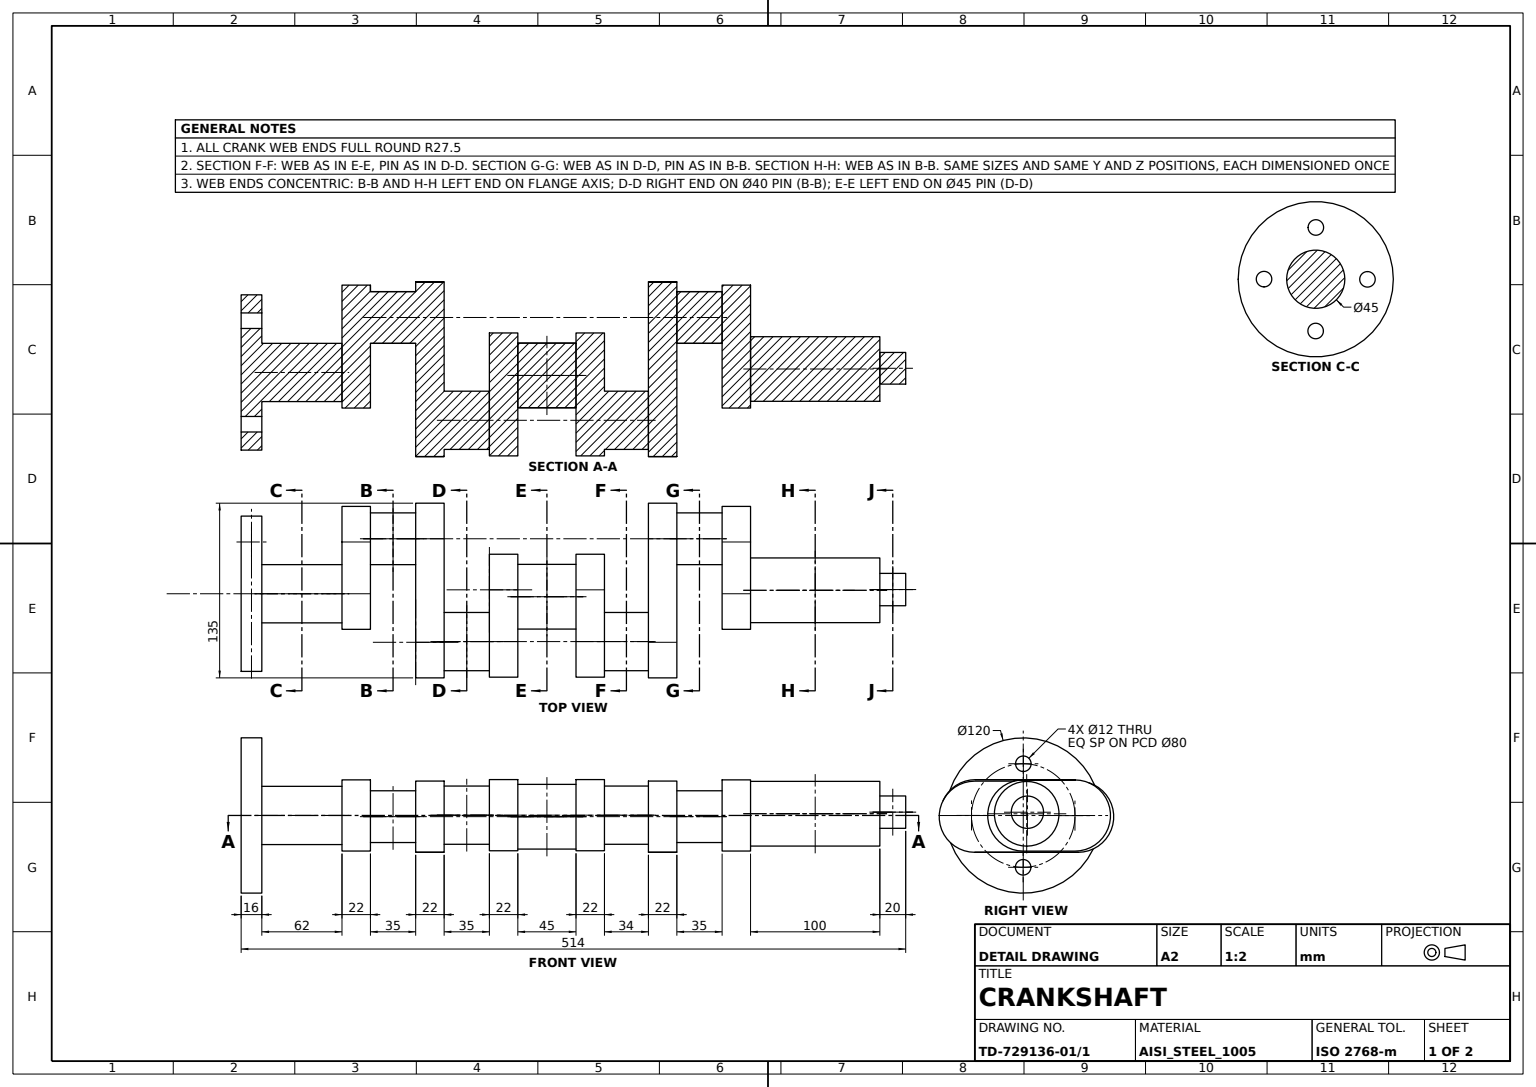
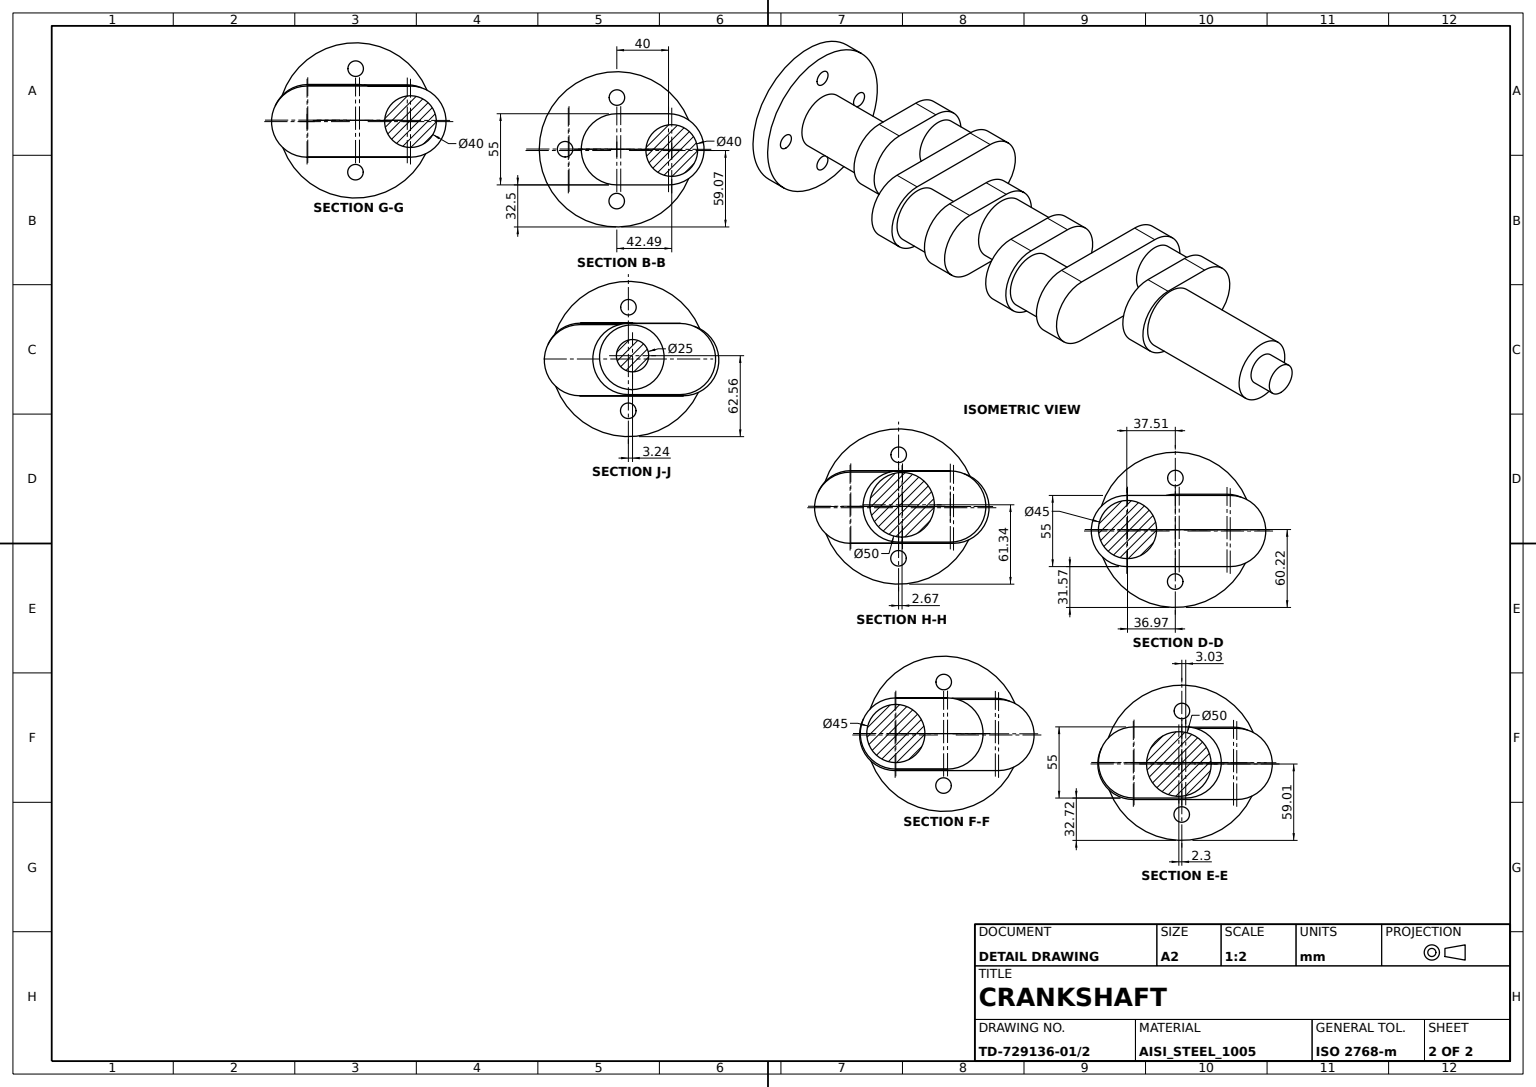
ISO-10303-21;
HEADER;
FILE_DESCRIPTION((''),'2;1');
FILE_NAME('','',(''),(''),'','','');
FILE_SCHEMA(('AUTOMOTIVE_DESIGN'));
ENDSEC;
DATA;
#1=APPLICATION_CONTEXT('');
#2=PRODUCT_CONTEXT('',#1,'mechanical');
#3=PRODUCT('','','',(#2));
#4=PRODUCT_DEFINITION_FORMATION('','',#3);
#5=PRODUCT_DEFINITION_CONTEXT('',#1,'design');
#6=PRODUCT_DEFINITION('','',#4,#5);
#7=PRODUCT_DEFINITION_SHAPE('','',#6);
#8=(LENGTH_UNIT()NAMED_UNIT(*)SI_UNIT(.MILLI.,.METRE.));
#9=(NAMED_UNIT(*)PLANE_ANGLE_UNIT()SI_UNIT($,.RADIAN.));
#10=(NAMED_UNIT(*)SI_UNIT($,.STERADIAN.)SOLID_ANGLE_UNIT());
#11=UNCERTAINTY_MEASURE_WITH_UNIT(LENGTH_MEASURE(0.005),#8,'distance_accuracy_value','');
#12=(GEOMETRIC_REPRESENTATION_CONTEXT(3)GLOBAL_UNCERTAINTY_ASSIGNED_CONTEXT((#11))GLOBAL_UNIT_ASSIGNED_CONTEXT((#8,#9,#10))REPRESENTATION_CONTEXT('',''));
#13=CARTESIAN_POINT('',(28.42745,-42.489879,-141.));
#14=VERTEX_POINT('',#13);
#15=CARTESIAN_POINT('',(-26.57255,-42.489879,-141.));
#16=VERTEX_POINT('',#15);
#17=CARTESIAN_POINT('',(0.92745,-42.489879,-141.));
#18=DIRECTION('',(0.,0.,-1.));
#19=DIRECTION('',(1.,0.,0.));
#20=AXIS2_PLACEMENT_3D('',#17,#18,#19);
#21=CIRCLE('',#20,27.5);
#22=EDGE_CURVE('',#14,#16,#21,.T.);
#23=ORIENTED_EDGE('',*,*,#22,.F.);
#24=CARTESIAN_POINT('',(28.42745,-42.489879,-119.));
#25=VERTEX_POINT('',#24);
#26=DIRECTION('',(0.,0.,1.));
#27=VECTOR('',#26,1000.);
#28=LINE('',#13,#27);
#29=EDGE_CURVE('',#14,#25,#28,.T.);
#30=ORIENTED_EDGE('',*,*,#29,.T.);
#31=CARTESIAN_POINT('',(-26.57255,-42.489879,-119.));
#32=VERTEX_POINT('',#31);
#33=CARTESIAN_POINT('',(0.92745,-42.489879,-119.));
#34=AXIS2_PLACEMENT_3D('',#33,#18,#19);
#35=CIRCLE('',#34,27.5);
#36=EDGE_CURVE('',#25,#32,#35,.T.);
#37=ORIENTED_EDGE('',*,*,#36,.T.);
#38=LINE('',#15,#27);
#39=EDGE_CURVE('',#16,#32,#38,.T.);
#40=ORIENTED_EDGE('',*,*,#39,.F.);
#41=EDGE_LOOP('',(#23,#30,#37,#40));
#42=FACE_BOUND('',#41,.T.);
#43=AXIS2_PLACEMENT_3D('',#17,#26,#19);
#44=CYLINDRICAL_SURFACE('',#43,27.5);
#45=ADVANCED_FACE('',(#42),#44,.T.);
#46=CARTESIAN_POINT('',(-26.57255,37.510121,-141.));
#47=VERTEX_POINT('',#46);
#48=CARTESIAN_POINT('',(-26.57255,37.510121,-119.));
#49=VERTEX_POINT('',#48);
#50=LINE('',#46,#27);
#51=EDGE_CURVE('',#47,#49,#50,.T.);
#52=ORIENTED_EDGE('',*,*,#51,.F.);
#53=DIRECTION('',(0.,1.,0.));
#54=VECTOR('',#53,1000.);
#55=LINE('',#15,#54);
#56=EDGE_CURVE('',#16,#47,#55,.T.);
#57=ORIENTED_EDGE('',*,*,#56,.F.);
#58=ORIENTED_EDGE('',*,*,#39,.T.);
#59=LINE('',#31,#54);
#60=EDGE_CURVE('',#32,#49,#59,.T.);
#61=ORIENTED_EDGE('',*,*,#60,.T.);
#62=EDGE_LOOP('',(#52,#57,#58,#61));
#63=FACE_BOUND('',#62,.T.);
#64=AXIS2_PLACEMENT_3D('',#15,#19,#53);
#65=PLANE('',#64);
#66=ADVANCED_FACE('',(#63),#65,.F.);
#67=ORIENTED_EDGE('',*,*,#29,.F.);
#68=CARTESIAN_POINT('',(28.42745,37.510121,-141.));
#69=VERTEX_POINT('',#68);
#70=DIRECTION('',(0.,-1.,0.));
#71=VECTOR('',#70,1000.);
#72=LINE('',#68,#71);
#73=EDGE_CURVE('',#69,#14,#72,.T.);
#74=ORIENTED_EDGE('',*,*,#73,.F.);
#75=CARTESIAN_POINT('',(28.42745,37.510121,-119.));
#76=VERTEX_POINT('',#75);
#77=LINE('',#68,#27);
#78=EDGE_CURVE('',#69,#76,#77,.T.);
#79=ORIENTED_EDGE('',*,*,#78,.T.);
#80=LINE('',#75,#71);
#81=EDGE_CURVE('',#76,#25,#80,.T.);
#82=ORIENTED_EDGE('',*,*,#81,.T.);
#83=EDGE_LOOP('',(#67,#74,#79,#82));
#84=FACE_BOUND('',#83,.T.);
#85=DIRECTION('',(-1.,0.,0.));
#86=AXIS2_PLACEMENT_3D('',#68,#85,#70);
#87=PLANE('',#86);
#88=ADVANCED_FACE('',(#84),#87,.F.);
#89=CARTESIAN_POINT('',(22.280438,36.967084,-176.));
#90=VERTEX_POINT('',#89);
#91=CARTESIAN_POINT('',(-0.219562,36.967084,-176.));
#92=AXIS2_PLACEMENT_3D('',#91,#18,#19);
#93=CIRCLE('',#92,22.5);
#94=EDGE_CURVE('',#90,#90,#93,.T.);
#95=ORIENTED_EDGE('',*,*,#94,.F.);
#96=EDGE_LOOP('',(#95));
#97=FACE_BOUND('',#96,.T.);
#98=CARTESIAN_POINT('',(22.280438,36.967084,-141.));
#99=VERTEX_POINT('',#98);
#100=CARTESIAN_POINT('',(-0.219562,36.967084,-141.));
#101=AXIS2_PLACEMENT_3D('',#100,#18,#19);
#102=CIRCLE('',#101,22.5);
#103=EDGE_CURVE('',#99,#99,#102,.T.);
#104=ORIENTED_EDGE('',*,*,#103,.T.);
#105=EDGE_LOOP('',(#104));
#106=FACE_BOUND('',#105,.T.);
#107=AXIS2_PLACEMENT_3D('',#91,#26,#19);
#108=CYLINDRICAL_SURFACE('',#107,22.5);
#109=ADVANCED_FACE('',(#97,#106),#108,.T.);
#110=CARTESIAN_POINT('',(20.92745,-42.489879,-84.));
#111=VERTEX_POINT('',#110);
#112=CARTESIAN_POINT('',(0.92745,-42.489879,-84.));
#113=AXIS2_PLACEMENT_3D('',#112,#18,#19);
#114=CIRCLE('',#113,20.);
#115=EDGE_CURVE('',#111,#111,#114,.T.);
#116=ORIENTED_EDGE('',*,*,#115,.T.);
#117=EDGE_LOOP('',(#116));
#118=FACE_BOUND('',#117,.T.);
#119=CARTESIAN_POINT('',(20.92745,-42.489879,-119.));
#120=VERTEX_POINT('',#119);
#121=CIRCLE('',#34,20.);
#122=EDGE_CURVE('',#120,#120,#121,.T.);
#123=ORIENTED_EDGE('',*,*,#122,.F.);
#124=EDGE_LOOP('',(#123));
#125=FACE_BOUND('',#124,.T.);
#126=AXIS2_PLACEMENT_3D('',#33,#26,#19);
#127=CYLINDRICAL_SURFACE('',#126,20.);
#128=ADVANCED_FACE('',(#118,#125),#127,.T.);
#129=ORIENTED_EDGE('',*,*,#122,.T.);
#130=EDGE_LOOP('',(#129));
#131=FACE_BOUND('',#130,.T.);
#132=CARTESIAN_POINT('',(0.92745,37.510121,-119.));
#133=AXIS2_PLACEMENT_3D('',#132,#18,#19);
#134=CIRCLE('',#133,27.5);
#135=EDGE_CURVE('',#49,#76,#134,.T.);
#136=ORIENTED_EDGE('',*,*,#135,.F.);
#137=ORIENTED_EDGE('',*,*,#60,.F.);
#138=ORIENTED_EDGE('',*,*,#36,.F.);
#139=ORIENTED_EDGE('',*,*,#81,.F.);
#140=EDGE_LOOP('',(#136,#137,#138,#139));
#141=FACE_BOUND('',#140,.T.);
#142=AXIS2_PLACEMENT_3D('',#132,#18,#85);
#143=PLANE('',#142);
#144=ADVANCED_FACE('',(#131,#141),#143,.F.);
#145=CARTESIAN_POINT('',(27.5,-40.,-62.));
#146=VERTEX_POINT('',#145);
#147=CARTESIAN_POINT('',(-27.5,-40.,-62.));
#148=VERTEX_POINT('',#147);
#149=CARTESIAN_POINT('',(0.,-40.,-62.));
#150=AXIS2_PLACEMENT_3D('',#149,#18,#53);
#151=CIRCLE('',#150,27.5);
#152=EDGE_CURVE('',#146,#148,#151,.T.);
#153=ORIENTED_EDGE('',*,*,#152,.F.);
#154=CARTESIAN_POINT('',(27.5,0.,-62.));
#155=VERTEX_POINT('',#154);
#156=LINE('',#154,#71);
#157=EDGE_CURVE('',#155,#146,#156,.T.);
#158=ORIENTED_EDGE('',*,*,#157,.F.);
#159=CARTESIAN_POINT('',(-27.5,0.,-62.));
#160=VERTEX_POINT('',#159);
#161=CARTESIAN_POINT('',(0.,0.,-62.));
#162=AXIS2_PLACEMENT_3D('',#161,#18,#53);
#163=CIRCLE('',#162,27.5);
#164=EDGE_CURVE('',#160,#155,#163,.T.);
#165=ORIENTED_EDGE('',*,*,#164,.F.);
#166=LINE('',#147,#54);
#167=EDGE_CURVE('',#148,#160,#166,.T.);
#168=ORIENTED_EDGE('',*,*,#167,.F.);
#169=EDGE_LOOP('',(#153,#158,#165,#168));
#170=FACE_BOUND('',#169,.T.);
#171=AXIS2_PLACEMENT_3D('',#161,#18,#85);
#172=PLANE('',#171);
#173=ADVANCED_FACE('',(#170),#172,.F.);
#174=CARTESIAN_POINT('',(27.5,-40.,-84.));
#175=VERTEX_POINT('',#174);
#176=CARTESIAN_POINT('',(-27.5,-40.,-84.));
#177=VERTEX_POINT('',#176);
#178=CARTESIAN_POINT('',(0.,-40.,-84.));
#179=AXIS2_PLACEMENT_3D('',#178,#18,#53);
#180=CIRCLE('',#179,27.5);
#181=EDGE_CURVE('',#175,#177,#180,.T.);
#182=ORIENTED_EDGE('',*,*,#181,.T.);
#183=CARTESIAN_POINT('',(-27.5,0.,-84.));
#184=VERTEX_POINT('',#183);
#185=LINE('',#176,#54);
#186=EDGE_CURVE('',#177,#184,#185,.T.);
#187=ORIENTED_EDGE('',*,*,#186,.T.);
#188=CARTESIAN_POINT('',(27.5,0.,-84.));
#189=VERTEX_POINT('',#188);
#190=CARTESIAN_POINT('',(0.,0.,-84.));
#191=AXIS2_PLACEMENT_3D('',#190,#18,#53);
#192=CIRCLE('',#191,27.5);
#193=EDGE_CURVE('',#184,#189,#192,.T.);
#194=ORIENTED_EDGE('',*,*,#193,.T.);
#195=LINE('',#188,#71);
#196=EDGE_CURVE('',#189,#175,#195,.T.);
#197=ORIENTED_EDGE('',*,*,#196,.T.);
#198=EDGE_LOOP('',(#182,#187,#194,#197));
#199=FACE_BOUND('',#198,.T.);
#200=ORIENTED_EDGE('',*,*,#115,.F.);
#201=EDGE_LOOP('',(#200));
#202=FACE_BOUND('',#201,.T.);
#203=AXIS2_PLACEMENT_3D('',#190,#18,#85);
#204=PLANE('',#203);
#205=ADVANCED_FACE('',(#199,#202),#204,.T.);
#206=ORIENTED_EDGE('',*,*,#164,.T.);
#207=LINE('',#188,#27);
#208=EDGE_CURVE('',#189,#155,#207,.T.);
#209=ORIENTED_EDGE('',*,*,#208,.F.);
#210=ORIENTED_EDGE('',*,*,#193,.F.);
#211=LINE('',#183,#27);
#212=EDGE_CURVE('',#184,#160,#211,.T.);
#213=ORIENTED_EDGE('',*,*,#212,.T.);
#214=EDGE_LOOP('',(#206,#209,#210,#213));
#215=FACE_BOUND('',#214,.T.);
#216=AXIS2_PLACEMENT_3D('',#190,#26,#19);
#217=CYLINDRICAL_SURFACE('',#216,27.5);
#218=ADVANCED_FACE('',(#215),#217,.T.);
#219=ORIENTED_EDGE('',*,*,#212,.F.);
#220=ORIENTED_EDGE('',*,*,#186,.F.);
#221=LINE('',#176,#27);
#222=EDGE_CURVE('',#177,#148,#221,.T.);
#223=ORIENTED_EDGE('',*,*,#222,.T.);
#224=ORIENTED_EDGE('',*,*,#167,.T.);
#225=EDGE_LOOP('',(#219,#220,#223,#224));
#226=FACE_BOUND('',#225,.T.);
#227=AXIS2_PLACEMENT_3D('',#176,#19,#18);
#228=PLANE('',#227);
#229=ADVANCED_FACE('',(#226),#228,.F.);
#230=LINE('',#174,#27);
#231=EDGE_CURVE('',#175,#146,#230,.T.);
#232=ORIENTED_EDGE('',*,*,#231,.F.);
#233=ORIENTED_EDGE('',*,*,#196,.F.);
#234=ORIENTED_EDGE('',*,*,#208,.T.);
#235=ORIENTED_EDGE('',*,*,#157,.T.);
#236=EDGE_LOOP('',(#232,#233,#234,#235));
#237=FACE_BOUND('',#236,.T.);
#238=AXIS2_PLACEMENT_3D('',#188,#85,#26);
#239=PLANE('',#238);
#240=ADVANCED_FACE('',(#237),#239,.F.);
#241=ORIENTED_EDGE('',*,*,#94,.T.);
#242=EDGE_LOOP('',(#241));
#243=FACE_BOUND('',#242,.T.);
#244=AXIS2_PLACEMENT_3D('',#91,#18,#85);
#245=PLANE('',#244);
#246=ADVANCED_FACE('',(#243),#245,.T.);
#247=ORIENTED_EDGE('',*,*,#152,.T.);
#248=ORIENTED_EDGE('',*,*,#222,.F.);
#249=ORIENTED_EDGE('',*,*,#181,.F.);
#250=ORIENTED_EDGE('',*,*,#231,.T.);
#251=EDGE_LOOP('',(#247,#248,#249,#250));
#252=FACE_BOUND('',#251,.T.);
#253=AXIS2_PLACEMENT_3D('',#178,#26,#19);
#254=CYLINDRICAL_SURFACE('',#253,27.5);
#255=ADVANCED_FACE('',(#252),#254,.T.);
#256=CARTESIAN_POINT('',(0.92745,37.510121,-141.));
#257=AXIS2_PLACEMENT_3D('',#256,#18,#19);
#258=CIRCLE('',#257,27.5);
#259=EDGE_CURVE('',#47,#69,#258,.T.);
#260=ORIENTED_EDGE('',*,*,#259,.F.);
#261=ORIENTED_EDGE('',*,*,#51,.T.);
#262=ORIENTED_EDGE('',*,*,#135,.T.);
#263=ORIENTED_EDGE('',*,*,#78,.F.);
#264=EDGE_LOOP('',(#260,#261,#262,#263));
#265=FACE_BOUND('',#264,.T.);
#266=AXIS2_PLACEMENT_3D('',#256,#26,#19);
#267=CYLINDRICAL_SURFACE('',#266,27.5);
#268=ADVANCED_FACE('',(#265),#267,.T.);
#269=ORIENTED_EDGE('',*,*,#22,.T.);
#270=ORIENTED_EDGE('',*,*,#56,.T.);
#271=ORIENTED_EDGE('',*,*,#259,.T.);
#272=ORIENTED_EDGE('',*,*,#73,.T.);
#273=EDGE_LOOP('',(#269,#270,#271,#272));
#274=FACE_BOUND('',#273,.T.);
#275=ORIENTED_EDGE('',*,*,#103,.F.);
#276=EDGE_LOOP('',(#275));
#277=FACE_BOUND('',#276,.T.);
#278=AXIS2_PLACEMENT_3D('',#256,#18,#85);
#279=PLANE('',#278);
#280=ADVANCED_FACE('',(#274,#277),#279,.T.);
#281=CLOSED_SHELL('',(#45,#66,#88,#109,#128,#144,#173,#205,#218,#229,#240,#246,#255,#268,#280));
#282=MANIFOLD_SOLID_BREP('',#281);
#283=CARTESIAN_POINT('',(23.658853,-2.674928,-478.));
#284=VERTEX_POINT('',#283);
#285=CARTESIAN_POINT('',(-1.341147,-2.674928,-478.));
#286=AXIS2_PLACEMENT_3D('',#285,#18,#19);
#287=CIRCLE('',#286,25.);
#288=EDGE_CURVE('',#284,#284,#287,.T.);
#289=ORIENTED_EDGE('',*,*,#288,.F.);
#290=EDGE_LOOP('',(#289));
#291=FACE_BOUND('',#290,.T.);
#292=CARTESIAN_POINT('',(23.658853,-2.674928,-378.));
#293=VERTEX_POINT('',#292);
#294=CARTESIAN_POINT('',(-1.341147,-2.674928,-378.));
#295=AXIS2_PLACEMENT_3D('',#294,#18,#19);
#296=CIRCLE('',#295,25.);
#297=EDGE_CURVE('',#293,#293,#296,.T.);
#298=ORIENTED_EDGE('',*,*,#297,.T.);
#299=EDGE_LOOP('',(#298));
#300=FACE_BOUND('',#299,.T.);
#301=AXIS2_PLACEMENT_3D('',#285,#26,#19);
#302=CYLINDRICAL_SURFACE('',#301,25.);
#303=ADVANCED_FACE('',(#291,#300),#302,.T.);
#304=ORIENTED_EDGE('',*,*,#297,.F.);
#305=EDGE_LOOP('',(#304));
#306=FACE_BOUND('',#305,.T.);
#307=AXIS2_PLACEMENT_3D('',#294,#18,#85);
#308=PLANE('',#307);
#309=ADVANCED_FACE('',(#306),#308,.F.);
#310=ORIENTED_EDGE('',*,*,#288,.T.);
#311=EDGE_LOOP('',(#310));
#312=FACE_BOUND('',#311,.T.);
#313=AXIS2_PLACEMENT_3D('',#285,#18,#85);
#314=PLANE('',#313);
#315=ADVANCED_FACE('',(#312),#314,.T.);
#316=CLOSED_SHELL('',(#303,#309,#315));
#317=MANIFOLD_SOLID_BREP('',#316);
#318=CARTESIAN_POINT('',(9.940539,-3.236305,-478.));
#319=VERTEX_POINT('',#318);
#320=CARTESIAN_POINT('',(-2.559461,-3.236305,-478.));
#321=AXIS2_PLACEMENT_3D('',#320,#18,#19);
#322=CIRCLE('',#321,12.5);
#323=EDGE_CURVE('',#319,#319,#322,.T.);
#324=ORIENTED_EDGE('',*,*,#323,.F.);
#325=EDGE_LOOP('',(#324));
#326=FACE_BOUND('',#325,.T.);
#327=AXIS2_PLACEMENT_3D('',#320,#18,#85);
#328=PLANE('',#327);
#329=ADVANCED_FACE('',(#326),#328,.F.);
#330=ORIENTED_EDGE('',*,*,#323,.T.);
#331=EDGE_LOOP('',(#330));
#332=FACE_BOUND('',#331,.T.);
#333=CARTESIAN_POINT('',(9.940539,-3.236305,-498.));
#334=VERTEX_POINT('',#333);
#335=CARTESIAN_POINT('',(-2.559461,-3.236305,-498.));
#336=AXIS2_PLACEMENT_3D('',#335,#18,#19);
#337=CIRCLE('',#336,12.5);
#338=EDGE_CURVE('',#334,#334,#337,.T.);
#339=ORIENTED_EDGE('',*,*,#338,.F.);
#340=EDGE_LOOP('',(#339));
#341=FACE_BOUND('',#340,.T.);
#342=AXIS2_PLACEMENT_3D('',#335,#26,#19);
#343=CYLINDRICAL_SURFACE('',#342,12.5);
#344=ADVANCED_FACE('',(#332,#341),#343,.T.);
#345=ORIENTED_EDGE('',*,*,#338,.T.);
#346=EDGE_LOOP('',(#345));
#347=FACE_BOUND('',#346,.T.);
#348=AXIS2_PLACEMENT_3D('',#335,#18,#85);
#349=PLANE('',#348);
#350=ADVANCED_FACE('',(#347),#349,.T.);
#351=CLOSED_SHELL('',(#329,#344,#350));
#352=MANIFOLD_SOLID_BREP('',#351);
#353=CARTESIAN_POINT('',(-39.999919,5.919571,0.));
#354=VERTEX_POINT('',#353);
#355=CARTESIAN_POINT('',(-39.999919,-0.080429,0.));
#356=AXIS2_PLACEMENT_3D('',#355,#26,#53);
#357=CIRCLE('',#356,6.);
#358=EDGE_CURVE('',#354,#354,#357,.T.);
#359=ORIENTED_EDGE('',*,*,#358,.F.);
#360=EDGE_LOOP('',(#359));
#361=FACE_BOUND('',#360,.T.);
#362=CARTESIAN_POINT('',(-39.999919,5.919571,16.));
#363=VERTEX_POINT('',#362);
#364=CARTESIAN_POINT('',(-39.999919,-0.080429,16.));
#365=AXIS2_PLACEMENT_3D('',#364,#26,#53);
#366=CIRCLE('',#365,6.);
#367=EDGE_CURVE('',#363,#363,#366,.T.);
#368=ORIENTED_EDGE('',*,*,#367,.T.);
#369=EDGE_LOOP('',(#368));
#370=FACE_BOUND('',#369,.T.);
#371=AXIS2_PLACEMENT_3D('',#364,#18,#85);
#372=CYLINDRICAL_SURFACE('',#371,6.);
#373=ADVANCED_FACE('',(#361,#370),#372,.F.);
#374=CARTESIAN_POINT('',(39.999919,-5.919571,16.));
#375=VERTEX_POINT('',#374);
#376=CARTESIAN_POINT('',(39.999919,0.080429,16.));
#377=AXIS2_PLACEMENT_3D('',#376,#26,#70);
#378=CIRCLE('',#377,6.);
#379=EDGE_CURVE('',#375,#375,#378,.T.);
#380=ORIENTED_EDGE('',*,*,#379,.F.);
#381=EDGE_LOOP('',(#380));
#382=FACE_BOUND('',#381,.T.);
#383=CARTESIAN_POINT('',(5.919571,39.999919,16.));
#384=VERTEX_POINT('',#383);
#385=CARTESIAN_POINT('',(-0.080429,39.999919,16.));
#386=AXIS2_PLACEMENT_3D('',#385,#26,#19);
#387=CIRCLE('',#386,6.);
#388=EDGE_CURVE('',#384,#384,#387,.T.);
#389=ORIENTED_EDGE('',*,*,#388,.F.);
#390=EDGE_LOOP('',(#389));
#391=FACE_BOUND('',#390,.T.);
#392=CARTESIAN_POINT('',(-5.919571,-39.999919,16.));
#393=VERTEX_POINT('',#392);
#394=CARTESIAN_POINT('',(0.080429,-39.999919,16.));
#395=AXIS2_PLACEMENT_3D('',#394,#26,#85);
#396=CIRCLE('',#395,6.);
#397=EDGE_CURVE('',#393,#393,#396,.T.);
#398=ORIENTED_EDGE('',*,*,#397,.F.);
#399=EDGE_LOOP('',(#398));
#400=FACE_BOUND('',#399,.T.);
#401=CARTESIAN_POINT('',(0.,60.,16.));
#402=VERTEX_POINT('',#401);
#403=CARTESIAN_POINT('',(0.,0.,16.));
#404=AXIS2_PLACEMENT_3D('',#403,#26,#53);
#405=CIRCLE('',#404,60.);
#406=EDGE_CURVE('',#402,#402,#405,.T.);
#407=ORIENTED_EDGE('',*,*,#406,.T.);
#408=EDGE_LOOP('',(#407));
#409=FACE_BOUND('',#408,.T.);
#410=ORIENTED_EDGE('',*,*,#367,.F.);
#411=EDGE_LOOP('',(#410));
#412=FACE_BOUND('',#411,.T.);
#413=AXIS2_PLACEMENT_3D('',#403,#26,#19);
#414=PLANE('',#413);
#415=ADVANCED_FACE('',(#382,#391,#400,#409,#412),#414,.T.);
#416=CARTESIAN_POINT('',(-5.919571,-39.999919,0.));
#417=VERTEX_POINT('',#416);
#418=CARTESIAN_POINT('',(0.080429,-39.999919,0.));
#419=AXIS2_PLACEMENT_3D('',#418,#26,#85);
#420=CIRCLE('',#419,6.);
#421=EDGE_CURVE('',#417,#417,#420,.T.);
#422=ORIENTED_EDGE('',*,*,#421,.F.);
#423=EDGE_LOOP('',(#422));
#424=FACE_BOUND('',#423,.T.);
#425=ORIENTED_EDGE('',*,*,#397,.T.);
#426=EDGE_LOOP('',(#425));
#427=FACE_BOUND('',#426,.T.);
#428=AXIS2_PLACEMENT_3D('',#394,#18,#85);
#429=CYLINDRICAL_SURFACE('',#428,6.);
#430=ADVANCED_FACE('',(#424,#427),#429,.F.);
#431=CARTESIAN_POINT('',(0.,22.5,0.));
#432=VERTEX_POINT('',#431);
#433=CARTESIAN_POINT('',(0.,0.,0.));
#434=AXIS2_PLACEMENT_3D('',#433,#18,#53);
#435=CIRCLE('',#434,22.5);
#436=EDGE_CURVE('',#432,#432,#435,.T.);
#437=ORIENTED_EDGE('',*,*,#436,.T.);
#438=EDGE_LOOP('',(#437));
#439=FACE_BOUND('',#438,.T.);
#440=CARTESIAN_POINT('',(0.,22.5,-62.));
#441=VERTEX_POINT('',#440);
#442=CIRCLE('',#162,22.5);
#443=EDGE_CURVE('',#441,#441,#442,.T.);
#444=ORIENTED_EDGE('',*,*,#443,.F.);
#445=EDGE_LOOP('',(#444));
#446=FACE_BOUND('',#445,.T.);
#447=AXIS2_PLACEMENT_3D('',#161,#26,#19);
#448=CYLINDRICAL_SURFACE('',#447,22.5);
#449=ADVANCED_FACE('',(#439,#446),#448,.T.);
#450=CARTESIAN_POINT('',(5.919571,39.999919,0.));
#451=VERTEX_POINT('',#450);
#452=CARTESIAN_POINT('',(-0.080429,39.999919,0.));
#453=AXIS2_PLACEMENT_3D('',#452,#26,#19);
#454=CIRCLE('',#453,6.);
#455=EDGE_CURVE('',#451,#451,#454,.T.);
#456=ORIENTED_EDGE('',*,*,#455,.F.);
#457=EDGE_LOOP('',(#456));
#458=FACE_BOUND('',#457,.T.);
#459=ORIENTED_EDGE('',*,*,#388,.T.);
#460=EDGE_LOOP('',(#459));
#461=FACE_BOUND('',#460,.T.);
#462=AXIS2_PLACEMENT_3D('',#385,#18,#85);
#463=CYLINDRICAL_SURFACE('',#462,6.);
#464=ADVANCED_FACE('',(#458,#461),#463,.F.);
#465=CARTESIAN_POINT('',(0.,60.,0.));
#466=VERTEX_POINT('',#465);
#467=AXIS2_PLACEMENT_3D('',#433,#26,#53);
#468=CIRCLE('',#467,60.);
#469=EDGE_CURVE('',#466,#466,#468,.T.);
#470=ORIENTED_EDGE('',*,*,#469,.T.);
#471=EDGE_LOOP('',(#470));
#472=FACE_BOUND('',#471,.T.);
#473=ORIENTED_EDGE('',*,*,#406,.F.);
#474=EDGE_LOOP('',(#473));
#475=FACE_BOUND('',#474,.T.);
#476=AXIS2_PLACEMENT_3D('',#403,#18,#85);
#477=CYLINDRICAL_SURFACE('',#476,60.);
#478=ADVANCED_FACE('',(#472,#475),#477,.T.);
#479=ORIENTED_EDGE('',*,*,#443,.T.);
#480=EDGE_LOOP('',(#479));
#481=FACE_BOUND('',#480,.T.);
#482=ADVANCED_FACE('',(#481),#172,.T.);
#483=CARTESIAN_POINT('',(39.999919,-5.919571,0.));
#484=VERTEX_POINT('',#483);
#485=CARTESIAN_POINT('',(39.999919,0.080429,0.));
#486=AXIS2_PLACEMENT_3D('',#485,#26,#70);
#487=CIRCLE('',#486,6.);
#488=EDGE_CURVE('',#484,#484,#487,.T.);
#489=ORIENTED_EDGE('',*,*,#488,.F.);
#490=EDGE_LOOP('',(#489));
#491=FACE_BOUND('',#490,.T.);
#492=ORIENTED_EDGE('',*,*,#379,.T.);
#493=EDGE_LOOP('',(#492));
#494=FACE_BOUND('',#493,.T.);
#495=AXIS2_PLACEMENT_3D('',#376,#18,#85);
#496=CYLINDRICAL_SURFACE('',#495,6.);
#497=ADVANCED_FACE('',(#491,#494),#496,.F.);
#498=ORIENTED_EDGE('',*,*,#469,.F.);
#499=EDGE_LOOP('',(#498));
#500=FACE_BOUND('',#499,.T.);
#501=ORIENTED_EDGE('',*,*,#358,.T.);
#502=EDGE_LOOP('',(#501));
#503=FACE_BOUND('',#502,.T.);
#504=ORIENTED_EDGE('',*,*,#455,.T.);
#505=EDGE_LOOP('',(#504));
#506=FACE_BOUND('',#505,.T.);
#507=ORIENTED_EDGE('',*,*,#436,.F.);
#508=EDGE_LOOP('',(#507));
#509=FACE_BOUND('',#508,.T.);
#510=ORIENTED_EDGE('',*,*,#488,.T.);
#511=EDGE_LOOP('',(#510));
#512=FACE_BOUND('',#511,.T.);
#513=ORIENTED_EDGE('',*,*,#421,.T.);
#514=EDGE_LOOP('',(#513));
#515=FACE_BOUND('',#514,.T.);
#516=AXIS2_PLACEMENT_3D('',#433,#26,#19);
#517=PLANE('',#516);
#518=ADVANCED_FACE('',(#500,#503,#506,#509,#512,#515),#517,.F.);
#519=CLOSED_SHELL('',(#373,#415,#430,#449,#464,#478,#482,#497,#518));
#520=MANIFOLD_SOLID_BREP('',#519);
#521=CARTESIAN_POINT('',(-27.719562,36.967084,-198.));
#522=VERTEX_POINT('',#521);
#523=CARTESIAN_POINT('',(-27.719562,36.967084,-176.));
#524=VERTEX_POINT('',#523);
#525=LINE('',#521,#27);
#526=EDGE_CURVE('',#522,#524,#525,.T.);
#527=ORIENTED_EDGE('',*,*,#526,.T.);
#528=CARTESIAN_POINT('',(27.280438,36.967084,-176.));
#529=VERTEX_POINT('',#528);
#530=CIRCLE('',#92,27.5);
#531=EDGE_CURVE('',#524,#529,#530,.T.);
#532=ORIENTED_EDGE('',*,*,#531,.T.);
#533=CARTESIAN_POINT('',(27.280438,36.967084,-198.));
#534=VERTEX_POINT('',#533);
#535=LINE('',#533,#27);
#536=EDGE_CURVE('',#534,#529,#535,.T.);
#537=ORIENTED_EDGE('',*,*,#536,.F.);
#538=CARTESIAN_POINT('',(-0.219562,36.967084,-198.));
#539=AXIS2_PLACEMENT_3D('',#538,#18,#19);
#540=CIRCLE('',#539,27.5);
#541=EDGE_CURVE('',#522,#534,#540,.T.);
#542=ORIENTED_EDGE('',*,*,#541,.F.);
#543=EDGE_LOOP('',(#527,#532,#537,#542));
#544=FACE_BOUND('',#543,.T.);
#545=AXIS2_PLACEMENT_3D('',#538,#26,#19);
#546=CYLINDRICAL_SURFACE('',#545,27.5);
#547=ADVANCED_FACE('',(#544),#546,.T.);
#548=ORIENTED_EDGE('',*,*,#541,.T.);
#549=CARTESIAN_POINT('',(27.280438,-3.032916,-198.));
#550=VERTEX_POINT('',#549);
#551=LINE('',#533,#71);
#552=EDGE_CURVE('',#534,#550,#551,.T.);
#553=ORIENTED_EDGE('',*,*,#552,.T.);
#554=CARTESIAN_POINT('',(-27.719562,-3.032916,-198.));
#555=VERTEX_POINT('',#554);
#556=CARTESIAN_POINT('',(-0.219562,-3.032916,-198.));
#557=AXIS2_PLACEMENT_3D('',#556,#18,#19);
#558=CIRCLE('',#557,27.5);
#559=EDGE_CURVE('',#550,#555,#558,.T.);
#560=ORIENTED_EDGE('',*,*,#559,.T.);
#561=LINE('',#554,#54);
#562=EDGE_CURVE('',#555,#522,#561,.T.);
#563=ORIENTED_EDGE('',*,*,#562,.T.);
#564=EDGE_LOOP('',(#548,#553,#560,#563));
#565=FACE_BOUND('',#564,.T.);
#566=AXIS2_PLACEMENT_3D('',#538,#18,#85);
#567=PLANE('',#566);
#568=ADVANCED_FACE('',(#565),#567,.T.);
#569=ORIENTED_EDGE('',*,*,#562,.F.);
#570=CARTESIAN_POINT('',(-27.719562,-3.032916,-176.));
#571=VERTEX_POINT('',#570);
#572=LINE('',#554,#27);
#573=EDGE_CURVE('',#555,#571,#572,.T.);
#574=ORIENTED_EDGE('',*,*,#573,.T.);
#575=LINE('',#570,#54);
#576=EDGE_CURVE('',#571,#524,#575,.T.);
#577=ORIENTED_EDGE('',*,*,#576,.T.);
#578=ORIENTED_EDGE('',*,*,#526,.F.);
#579=EDGE_LOOP('',(#569,#574,#577,#578));
#580=FACE_BOUND('',#579,.T.);
#581=AXIS2_PLACEMENT_3D('',#554,#19,#53);
#582=PLANE('',#581);
#583=ADVANCED_FACE('',(#580),#582,.F.);
#584=CARTESIAN_POINT('',(27.280438,-3.032916,-176.));
#585=VERTEX_POINT('',#584);
#586=CARTESIAN_POINT('',(-0.219562,-3.032916,-176.));
#587=AXIS2_PLACEMENT_3D('',#586,#18,#19);
#588=CIRCLE('',#587,27.5);
#589=EDGE_CURVE('',#585,#571,#588,.T.);
#590=ORIENTED_EDGE('',*,*,#589,.F.);
#591=LINE('',#528,#71);
#592=EDGE_CURVE('',#529,#585,#591,.T.);
#593=ORIENTED_EDGE('',*,*,#592,.F.);
#594=ORIENTED_EDGE('',*,*,#531,.F.);
#595=ORIENTED_EDGE('',*,*,#576,.F.);
#596=EDGE_LOOP('',(#590,#593,#594,#595));
#597=FACE_BOUND('',#596,.T.);
#598=ADVANCED_FACE('',(#597),#245,.F.);
#599=ORIENTED_EDGE('',*,*,#552,.F.);
#600=ORIENTED_EDGE('',*,*,#536,.T.);
#601=ORIENTED_EDGE('',*,*,#592,.T.);
#602=LINE('',#549,#27);
#603=EDGE_CURVE('',#550,#585,#602,.T.);
#604=ORIENTED_EDGE('',*,*,#603,.F.);
#605=EDGE_LOOP('',(#599,#600,#601,#604));
#606=FACE_BOUND('',#605,.T.);
#607=AXIS2_PLACEMENT_3D('',#533,#85,#26);
#608=PLANE('',#607);
#609=ADVANCED_FACE('',(#606),#608,.F.);
#610=ORIENTED_EDGE('',*,*,#603,.T.);
#611=ORIENTED_EDGE('',*,*,#589,.T.);
#612=ORIENTED_EDGE('',*,*,#573,.F.);
#613=ORIENTED_EDGE('',*,*,#559,.F.);
#614=EDGE_LOOP('',(#610,#611,#612,#613));
#615=FACE_BOUND('',#614,.T.);
#616=AXIS2_PLACEMENT_3D('',#556,#26,#19);
#617=CYLINDRICAL_SURFACE('',#616,27.5);
#618=ADVANCED_FACE('',(#615),#617,.T.);
#619=CLOSED_SHELL('',(#547,#568,#583,#598,#609,#618));
#620=MANIFOLD_SOLID_BREP('',#619);
#621=CARTESIAN_POINT('',(27.280438,-3.032916,-243.));
#622=VERTEX_POINT('',#621);
#623=CARTESIAN_POINT('',(27.280438,-3.032916,-265.));
#624=VERTEX_POINT('',#623);
#625=VECTOR('',#18,1000.);
#626=LINE('',#621,#625);
#627=EDGE_CURVE('',#622,#624,#626,.T.);
#628=ORIENTED_EDGE('',*,*,#627,.F.);
#629=CARTESIAN_POINT('',(-27.719562,-3.032916,-243.));
#630=VERTEX_POINT('',#629);
#631=CARTESIAN_POINT('',(-0.219562,-3.032916,-243.));
#632=AXIS2_PLACEMENT_3D('',#631,#18,#19);
#633=CIRCLE('',#632,27.5);
#634=EDGE_CURVE('',#622,#630,#633,.T.);
#635=ORIENTED_EDGE('',*,*,#634,.T.);
#636=CARTESIAN_POINT('',(-27.719562,-3.032916,-265.));
#637=VERTEX_POINT('',#636);
#638=LINE('',#629,#625);
#639=EDGE_CURVE('',#630,#637,#638,.T.);
#640=ORIENTED_EDGE('',*,*,#639,.T.);
#641=CARTESIAN_POINT('',(-0.219562,-3.032916,-265.));
#642=AXIS2_PLACEMENT_3D('',#641,#18,#19);
#643=CIRCLE('',#642,27.5);
#644=EDGE_CURVE('',#624,#637,#643,.T.);
#645=ORIENTED_EDGE('',*,*,#644,.F.);
#646=EDGE_LOOP('',(#628,#635,#640,#645));
#647=FACE_BOUND('',#646,.T.);
#648=AXIS2_PLACEMENT_3D('',#631,#18,#85);
#649=CYLINDRICAL_SURFACE('',#648,27.5);
#650=ADVANCED_FACE('',(#647),#649,.T.);
#651=CARTESIAN_POINT('',(22.280438,36.967084,-299.));
#652=VERTEX_POINT('',#651);
#653=CARTESIAN_POINT('',(-0.219562,36.967084,-299.));
#654=AXIS2_PLACEMENT_3D('',#653,#18,#19);
#655=CIRCLE('',#654,22.5);
#656=EDGE_CURVE('',#652,#652,#655,.T.);
#657=ORIENTED_EDGE('',*,*,#656,.F.);
#658=EDGE_LOOP('',(#657));
#659=FACE_BOUND('',#658,.T.);
#660=CARTESIAN_POINT('',(-22.719562,36.967084,-265.));
#661=VERTEX_POINT('',#660);
#662=CARTESIAN_POINT('',(-0.219562,36.967084,-265.));
#663=AXIS2_PLACEMENT_3D('',#662,#18,#85);
#664=CIRCLE('',#663,22.5);
#665=EDGE_CURVE('',#661,#661,#664,.F.);
#666=ORIENTED_EDGE('',*,*,#665,.F.);
#667=EDGE_LOOP('',(#666));
#668=FACE_BOUND('',#667,.T.);
#669=CARTESIAN_POINT('',(-0.219562,36.967084,-264.));
#670=AXIS2_PLACEMENT_3D('',#669,#18,#85);
#671=CYLINDRICAL_SURFACE('',#670,22.5);
#672=ADVANCED_FACE('',(#659,#668),#671,.T.);
#673=CARTESIAN_POINT('',(-27.719562,36.967084,-243.));
#674=VERTEX_POINT('',#673);
#675=LINE('',#629,#54);
#676=EDGE_CURVE('',#630,#674,#675,.T.);
#677=ORIENTED_EDGE('',*,*,#676,.T.);
#678=CARTESIAN_POINT('',(-27.719562,36.967084,-265.));
#679=VERTEX_POINT('',#678);
#680=LINE('',#673,#625);
#681=EDGE_CURVE('',#674,#679,#680,.T.);
#682=ORIENTED_EDGE('',*,*,#681,.T.);
#683=LINE('',#636,#54);
#684=EDGE_CURVE('',#637,#679,#683,.T.);
#685=ORIENTED_EDGE('',*,*,#684,.F.);
#686=ORIENTED_EDGE('',*,*,#639,.F.);
#687=EDGE_LOOP('',(#677,#682,#685,#686));
#688=FACE_BOUND('',#687,.T.);
#689=AXIS2_PLACEMENT_3D('',#629,#85,#70);
#690=PLANE('',#689);
#691=ADVANCED_FACE('',(#688),#690,.T.);
#692=CARTESIAN_POINT('',(27.280438,36.967084,-243.));
#693=VERTEX_POINT('',#692);
#694=LINE('',#692,#71);
#695=EDGE_CURVE('',#693,#622,#694,.T.);
#696=ORIENTED_EDGE('',*,*,#695,.T.);
#697=ORIENTED_EDGE('',*,*,#627,.T.);
#698=CARTESIAN_POINT('',(27.280438,36.967084,-265.));
#699=VERTEX_POINT('',#698);
#700=LINE('',#698,#71);
#701=EDGE_CURVE('',#699,#624,#700,.T.);
#702=ORIENTED_EDGE('',*,*,#701,.F.);
#703=LINE('',#692,#625);
#704=EDGE_CURVE('',#693,#699,#703,.T.);
#705=ORIENTED_EDGE('',*,*,#704,.F.);
#706=EDGE_LOOP('',(#696,#697,#702,#705));
#707=FACE_BOUND('',#706,.T.);
#708=AXIS2_PLACEMENT_3D('',#692,#19,#18);
#709=PLANE('',#708);
#710=ADVANCED_FACE('',(#707),#709,.T.);
#711=ORIENTED_EDGE('',*,*,#665,.T.);
#712=EDGE_LOOP('',(#711));
#713=FACE_BOUND('',#712,.T.);
#714=ORIENTED_EDGE('',*,*,#644,.T.);
#715=ORIENTED_EDGE('',*,*,#684,.T.);
#716=AXIS2_PLACEMENT_3D('',#662,#18,#19);
#717=CIRCLE('',#716,27.5);
#718=EDGE_CURVE('',#679,#699,#717,.T.);
#719=ORIENTED_EDGE('',*,*,#718,.T.);
#720=ORIENTED_EDGE('',*,*,#701,.T.);
#721=EDGE_LOOP('',(#714,#715,#719,#720));
#722=FACE_BOUND('',#721,.T.);
#723=PLANE('',#663);
#724=ADVANCED_FACE('',(#713,#722),#723,.T.);
#725=ORIENTED_EDGE('',*,*,#656,.T.);
#726=EDGE_LOOP('',(#725));
#727=FACE_BOUND('',#726,.T.);
#728=AXIS2_PLACEMENT_3D('',#653,#18,#85);
#729=PLANE('',#728);
#730=ADVANCED_FACE('',(#727),#729,.T.);
#731=ORIENTED_EDGE('',*,*,#676,.F.);
#732=ORIENTED_EDGE('',*,*,#634,.F.);
#733=ORIENTED_EDGE('',*,*,#695,.F.);
#734=CARTESIAN_POINT('',(-0.219562,36.967084,-243.));
#735=AXIS2_PLACEMENT_3D('',#734,#18,#19);
#736=CIRCLE('',#735,27.5);
#737=EDGE_CURVE('',#674,#693,#736,.T.);
#738=ORIENTED_EDGE('',*,*,#737,.F.);
#739=EDGE_LOOP('',(#731,#732,#733,#738));
#740=FACE_BOUND('',#739,.T.);
#741=AXIS2_PLACEMENT_3D('',#734,#18,#85);
#742=PLANE('',#741);
#743=ADVANCED_FACE('',(#740),#742,.F.);
#744=ORIENTED_EDGE('',*,*,#681,.F.);
#745=ORIENTED_EDGE('',*,*,#737,.T.);
#746=ORIENTED_EDGE('',*,*,#704,.T.);
#747=ORIENTED_EDGE('',*,*,#718,.F.);
#748=EDGE_LOOP('',(#744,#745,#746,#747));
#749=FACE_BOUND('',#748,.T.);
#750=CYLINDRICAL_SURFACE('',#741,27.5);
#751=ADVANCED_FACE('',(#749),#750,.T.);
#752=CLOSED_SHELL('',(#650,#672,#691,#710,#724,#730,#743,#751));
#753=MANIFOLD_SOLID_BREP('',#752);
#754=CARTESIAN_POINT('',(27.5,0.,-378.));
#755=VERTEX_POINT('',#754);
#756=CARTESIAN_POINT('',(27.5,-40.,-378.));
#757=VERTEX_POINT('',#756);
#758=LINE('',#754,#71);
#759=EDGE_CURVE('',#755,#757,#758,.T.);
#760=ORIENTED_EDGE('',*,*,#759,.T.);
#761=CARTESIAN_POINT('',(-27.5,-40.,-378.));
#762=VERTEX_POINT('',#761);
#763=CARTESIAN_POINT('',(0.,-40.,-378.));
#764=AXIS2_PLACEMENT_3D('',#763,#18,#53);
#765=CIRCLE('',#764,27.5);
#766=EDGE_CURVE('',#757,#762,#765,.T.);
#767=ORIENTED_EDGE('',*,*,#766,.T.);
#768=CARTESIAN_POINT('',(-27.5,0.,-378.));
#769=VERTEX_POINT('',#768);
#770=LINE('',#761,#54);
#771=EDGE_CURVE('',#762,#769,#770,.T.);
#772=ORIENTED_EDGE('',*,*,#771,.T.);
#773=CARTESIAN_POINT('',(0.,0.,-378.));
#774=AXIS2_PLACEMENT_3D('',#773,#18,#53);
#775=CIRCLE('',#774,27.5);
#776=EDGE_CURVE('',#769,#755,#775,.T.);
#777=ORIENTED_EDGE('',*,*,#776,.T.);
#778=EDGE_LOOP('',(#760,#767,#772,#777));
#779=FACE_BOUND('',#778,.T.);
#780=AXIS2_PLACEMENT_3D('',#773,#18,#85);
#781=PLANE('',#780);
#782=ADVANCED_FACE('',(#779),#781,.T.);
#783=CARTESIAN_POINT('',(27.5,-40.,-356.));
#784=VERTEX_POINT('',#783);
#785=LINE('',#783,#625);
#786=EDGE_CURVE('',#784,#757,#785,.T.);
#787=ORIENTED_EDGE('',*,*,#786,.F.);
#788=CARTESIAN_POINT('',(-27.5,-40.,-356.));
#789=VERTEX_POINT('',#788);
#790=CARTESIAN_POINT('',(0.,-40.,-356.));
#791=AXIS2_PLACEMENT_3D('',#790,#18,#53);
#792=CIRCLE('',#791,27.5);
#793=EDGE_CURVE('',#784,#789,#792,.T.);
#794=ORIENTED_EDGE('',*,*,#793,.T.);
#795=LINE('',#788,#625);
#796=EDGE_CURVE('',#789,#762,#795,.T.);
#797=ORIENTED_EDGE('',*,*,#796,.T.);
#798=ORIENTED_EDGE('',*,*,#766,.F.);
#799=EDGE_LOOP('',(#787,#794,#797,#798));
#800=FACE_BOUND('',#799,.T.);
#801=AXIS2_PLACEMENT_3D('',#790,#18,#85);
#802=CYLINDRICAL_SURFACE('',#801,27.5);
#803=ADVANCED_FACE('',(#800),#802,.T.);
#804=CARTESIAN_POINT('',(-27.5,0.,-356.));
#805=VERTEX_POINT('',#804);
#806=LINE('',#804,#625);
#807=EDGE_CURVE('',#805,#769,#806,.T.);
#808=ORIENTED_EDGE('',*,*,#807,.F.);
#809=CARTESIAN_POINT('',(27.5,0.,-356.));
#810=VERTEX_POINT('',#809);
#811=CARTESIAN_POINT('',(0.,0.,-356.));
#812=AXIS2_PLACEMENT_3D('',#811,#18,#53);
#813=CIRCLE('',#812,27.5);
#814=EDGE_CURVE('',#805,#810,#813,.T.);
#815=ORIENTED_EDGE('',*,*,#814,.T.);
#816=LINE('',#809,#625);
#817=EDGE_CURVE('',#810,#755,#816,.T.);
#818=ORIENTED_EDGE('',*,*,#817,.T.);
#819=ORIENTED_EDGE('',*,*,#776,.F.);
#820=EDGE_LOOP('',(#808,#815,#818,#819));
#821=FACE_BOUND('',#820,.T.);
#822=AXIS2_PLACEMENT_3D('',#811,#18,#85);
#823=CYLINDRICAL_SURFACE('',#822,27.5);
#824=ADVANCED_FACE('',(#821),#823,.T.);
#825=LINE('',#809,#71);
#826=EDGE_CURVE('',#810,#784,#825,.T.);
#827=ORIENTED_EDGE('',*,*,#826,.F.);
#828=ORIENTED_EDGE('',*,*,#814,.F.);
#829=LINE('',#788,#54);
#830=EDGE_CURVE('',#789,#805,#829,.T.);
#831=ORIENTED_EDGE('',*,*,#830,.F.);
#832=ORIENTED_EDGE('',*,*,#793,.F.);
#833=EDGE_LOOP('',(#827,#828,#831,#832));
#834=FACE_BOUND('',#833,.T.);
#835=PLANE('',#822);
#836=ADVANCED_FACE('',(#834),#835,.F.);
#837=ORIENTED_EDGE('',*,*,#796,.F.);
#838=ORIENTED_EDGE('',*,*,#830,.T.);
#839=ORIENTED_EDGE('',*,*,#807,.T.);
#840=ORIENTED_EDGE('',*,*,#771,.F.);
#841=EDGE_LOOP('',(#837,#838,#839,#840));
#842=FACE_BOUND('',#841,.T.);
#843=AXIS2_PLACEMENT_3D('',#788,#85,#26);
#844=PLANE('',#843);
#845=ADVANCED_FACE('',(#842),#844,.T.);
#846=ORIENTED_EDGE('',*,*,#826,.T.);
#847=ORIENTED_EDGE('',*,*,#786,.T.);
#848=ORIENTED_EDGE('',*,*,#759,.F.);
#849=ORIENTED_EDGE('',*,*,#817,.F.);
#850=EDGE_LOOP('',(#846,#847,#848,#849));
#851=FACE_BOUND('',#850,.T.);
#852=AXIS2_PLACEMENT_3D('',#809,#19,#18);
#853=PLANE('',#852);
#854=ADVANCED_FACE('',(#851),#853,.T.);
#855=CLOSED_SHELL('',(#782,#803,#824,#836,#845,#854));
#856=MANIFOLD_SOLID_BREP('',#855);
#857=CARTESIAN_POINT('',(0.98528,-22.702344,-243.));
#858=VERTEX_POINT('',#857);
#859=CARTESIAN_POINT('',(0.98528,2.297656,-243.));
#860=AXIS2_PLACEMENT_3D('',#859,#18,#70);
#861=CIRCLE('',#860,25.);
#862=EDGE_CURVE('',#858,#858,#861,.T.);
#863=ORIENTED_EDGE('',*,*,#862,.T.);
#864=EDGE_LOOP('',(#863));
#865=FACE_BOUND('',#864,.T.);
#866=AXIS2_PLACEMENT_3D('',#859,#18,#85);
#867=PLANE('',#866);
#868=ADVANCED_FACE('',(#865),#867,.T.);
#869=ORIENTED_EDGE('',*,*,#862,.F.);
#870=EDGE_LOOP('',(#869));
#871=FACE_BOUND('',#870,.T.);
#872=CARTESIAN_POINT('',(0.98528,-22.702344,-198.));
#873=VERTEX_POINT('',#872);
#874=CARTESIAN_POINT('',(0.98528,2.297656,-198.));
#875=AXIS2_PLACEMENT_3D('',#874,#18,#70);
#876=CIRCLE('',#875,25.);
#877=EDGE_CURVE('',#873,#873,#876,.T.);
#878=ORIENTED_EDGE('',*,*,#877,.T.);
#879=EDGE_LOOP('',(#878));
#880=FACE_BOUND('',#879,.T.);
#881=CARTESIAN_POINT('',(0.98528,2.297656,-220.5));
#882=AXIS2_PLACEMENT_3D('',#881,#26,#19);
#883=CYLINDRICAL_SURFACE('',#882,25.);
#884=ADVANCED_FACE('',(#871,#880),#883,.T.);
#885=ORIENTED_EDGE('',*,*,#877,.F.);
#886=EDGE_LOOP('',(#885));
#887=FACE_BOUND('',#886,.T.);
#888=AXIS2_PLACEMENT_3D('',#874,#18,#85);
#889=PLANE('',#888);
#890=ADVANCED_FACE('',(#887),#889,.F.);
#891=CLOSED_SHELL('',(#868,#884,#890));
#892=MANIFOLD_SOLID_BREP('',#891);
#893=CARTESIAN_POINT('',(28.42745,-42.489879,-299.));
#894=VERTEX_POINT('',#893);
#895=CARTESIAN_POINT('',(28.42745,-42.489879,-321.));
#896=VERTEX_POINT('',#895);
#897=LINE('',#893,#625);
#898=EDGE_CURVE('',#894,#896,#897,.T.);
#899=ORIENTED_EDGE('',*,*,#898,.T.);
#900=CARTESIAN_POINT('',(28.42745,37.510121,-321.));
#901=VERTEX_POINT('',#900);
#902=LINE('',#900,#71);
#903=EDGE_CURVE('',#901,#896,#902,.T.);
#904=ORIENTED_EDGE('',*,*,#903,.F.);
#905=CARTESIAN_POINT('',(28.42745,37.510121,-299.));
#906=VERTEX_POINT('',#905);
#907=LINE('',#905,#625);
#908=EDGE_CURVE('',#906,#901,#907,.T.);
#909=ORIENTED_EDGE('',*,*,#908,.F.);
#910=LINE('',#905,#71);
#911=EDGE_CURVE('',#906,#894,#910,.T.);
#912=ORIENTED_EDGE('',*,*,#911,.T.);
#913=EDGE_LOOP('',(#899,#904,#909,#912));
#914=FACE_BOUND('',#913,.T.);
#915=AXIS2_PLACEMENT_3D('',#905,#19,#53);
#916=PLANE('',#915);
#917=ADVANCED_FACE('',(#914),#916,.T.);
#918=CARTESIAN_POINT('',(-26.57255,37.510121,-299.));
#919=VERTEX_POINT('',#918);
#920=CARTESIAN_POINT('',(-26.57255,37.510121,-321.));
#921=VERTEX_POINT('',#920);
#922=LINE('',#918,#625);
#923=EDGE_CURVE('',#919,#921,#922,.T.);
#924=ORIENTED_EDGE('',*,*,#923,.F.);
#925=CARTESIAN_POINT('',(0.92745,37.510121,-299.));
#926=AXIS2_PLACEMENT_3D('',#925,#18,#19);
#927=CIRCLE('',#926,27.5);
#928=EDGE_CURVE('',#919,#906,#927,.T.);
#929=ORIENTED_EDGE('',*,*,#928,.T.);
#930=ORIENTED_EDGE('',*,*,#908,.T.);
#931=CARTESIAN_POINT('',(0.92745,37.510121,-321.));
#932=AXIS2_PLACEMENT_3D('',#931,#18,#19);
#933=CIRCLE('',#932,27.5);
#934=EDGE_CURVE('',#921,#901,#933,.T.);
#935=ORIENTED_EDGE('',*,*,#934,.F.);
#936=EDGE_LOOP('',(#924,#929,#930,#935));
#937=FACE_BOUND('',#936,.T.);
#938=AXIS2_PLACEMENT_3D('',#925,#18,#85);
#939=CYLINDRICAL_SURFACE('',#938,27.5);
#940=ADVANCED_FACE('',(#937),#939,.T.);
#941=ORIENTED_EDGE('',*,*,#928,.F.);
#942=CARTESIAN_POINT('',(-26.57255,-42.489879,-299.));
#943=VERTEX_POINT('',#942);
#944=LINE('',#942,#54);
#945=EDGE_CURVE('',#943,#919,#944,.T.);
#946=ORIENTED_EDGE('',*,*,#945,.F.);
#947=CARTESIAN_POINT('',(0.92745,-42.489879,-299.));
#948=AXIS2_PLACEMENT_3D('',#947,#18,#19);
#949=CIRCLE('',#948,27.5);
#950=EDGE_CURVE('',#894,#943,#949,.T.);
#951=ORIENTED_EDGE('',*,*,#950,.F.);
#952=ORIENTED_EDGE('',*,*,#911,.F.);
#953=EDGE_LOOP('',(#941,#946,#951,#952));
#954=FACE_BOUND('',#953,.T.);
#955=PLANE('',#938);
#956=ADVANCED_FACE('',(#954),#955,.F.);
#957=CARTESIAN_POINT('',(-26.57255,-42.489879,-321.));
#958=VERTEX_POINT('',#957);
#959=LINE('',#957,#54);
#960=EDGE_CURVE('',#958,#921,#959,.T.);
#961=ORIENTED_EDGE('',*,*,#960,.T.);
#962=ORIENTED_EDGE('',*,*,#934,.T.);
#963=ORIENTED_EDGE('',*,*,#903,.T.);
#964=CARTESIAN_POINT('',(0.92745,-42.489879,-321.));
#965=AXIS2_PLACEMENT_3D('',#964,#18,#19);
#966=CIRCLE('',#965,27.5);
#967=EDGE_CURVE('',#896,#958,#966,.T.);
#968=ORIENTED_EDGE('',*,*,#967,.T.);
#969=EDGE_LOOP('',(#961,#962,#963,#968));
#970=FACE_BOUND('',#969,.T.);
#971=AXIS2_PLACEMENT_3D('',#931,#18,#85);
#972=PLANE('',#971);
#973=ADVANCED_FACE('',(#970),#972,.T.);
#974=ORIENTED_EDGE('',*,*,#898,.F.);
#975=ORIENTED_EDGE('',*,*,#950,.T.);
#976=LINE('',#942,#625);
#977=EDGE_CURVE('',#943,#958,#976,.T.);
#978=ORIENTED_EDGE('',*,*,#977,.T.);
#979=ORIENTED_EDGE('',*,*,#967,.F.);
#980=EDGE_LOOP('',(#974,#975,#978,#979));
#981=FACE_BOUND('',#980,.T.);
#982=AXIS2_PLACEMENT_3D('',#947,#18,#85);
#983=CYLINDRICAL_SURFACE('',#982,27.5);
#984=ADVANCED_FACE('',(#981),#983,.T.);
#985=ORIENTED_EDGE('',*,*,#977,.F.);
#986=ORIENTED_EDGE('',*,*,#945,.T.);
#987=ORIENTED_EDGE('',*,*,#923,.T.);
#988=ORIENTED_EDGE('',*,*,#960,.F.);
#989=EDGE_LOOP('',(#985,#986,#987,#988));
#990=FACE_BOUND('',#989,.T.);
#991=AXIS2_PLACEMENT_3D('',#942,#85,#70);
#992=PLANE('',#991);
#993=ADVANCED_FACE('',(#990),#992,.T.);
#994=CLOSED_SHELL('',(#917,#940,#956,#973,#984,#993));
#995=MANIFOLD_SOLID_BREP('',#994);
#996=CARTESIAN_POINT('',(20.92745,-42.489879,-321.));
#997=VERTEX_POINT('',#996);
#998=CIRCLE('',#965,20.);
#999=EDGE_CURVE('',#997,#997,#998,.T.);
#1000=ORIENTED_EDGE('',*,*,#999,.T.);
#1001=EDGE_LOOP('',(#1000));
#1002=FACE_BOUND('',#1001,.T.);
#1003=CARTESIAN_POINT('',(20.92745,-42.489879,-356.));
#1004=VERTEX_POINT('',#1003);
#1005=CARTESIAN_POINT('',(0.92745,-42.489879,-356.));
#1006=AXIS2_PLACEMENT_3D('',#1005,#18,#19);
#1007=CIRCLE('',#1006,20.);
#1008=EDGE_CURVE('',#1004,#1004,#1007,.T.);
#1009=ORIENTED_EDGE('',*,*,#1008,.F.);
#1010=EDGE_LOOP('',(#1009));
#1011=FACE_BOUND('',#1010,.T.);
#1012=AXIS2_PLACEMENT_3D('',#964,#18,#85);
#1013=CYLINDRICAL_SURFACE('',#1012,20.);
#1014=ADVANCED_FACE('',(#1002,#1011),#1013,.T.);
#1015=ORIENTED_EDGE('',*,*,#999,.F.);
#1016=EDGE_LOOP('',(#1015));
#1017=FACE_BOUND('',#1016,.T.);
#1018=PLANE('',#1012);
#1019=ADVANCED_FACE('',(#1017),#1018,.F.);
#1020=ORIENTED_EDGE('',*,*,#1008,.T.);
#1021=EDGE_LOOP('',(#1020));
#1022=FACE_BOUND('',#1021,.T.);
#1023=AXIS2_PLACEMENT_3D('',#1005,#18,#85);
#1024=PLANE('',#1023);
#1025=ADVANCED_FACE('',(#1022),#1024,.T.);
#1026=CLOSED_SHELL('',(#1014,#1019,#1025));
#1027=MANIFOLD_SOLID_BREP('',#1026);
#1028=ADVANCED_BREP_SHAPE_REPRESENTATION('',(#282,#317,#352,#520,#620,#753,#856,#892,#995,#1027),#12);
#1029=SHAPE_DEFINITION_REPRESENTATION(#7,#1028);
ENDSEC;
END-ISO-10303-21;
